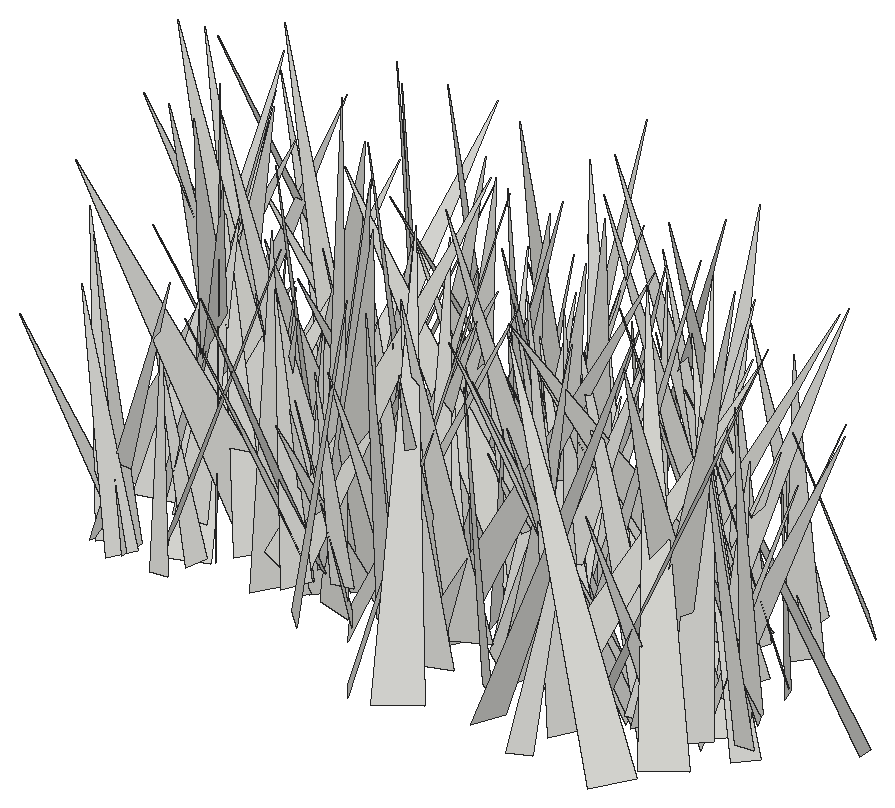
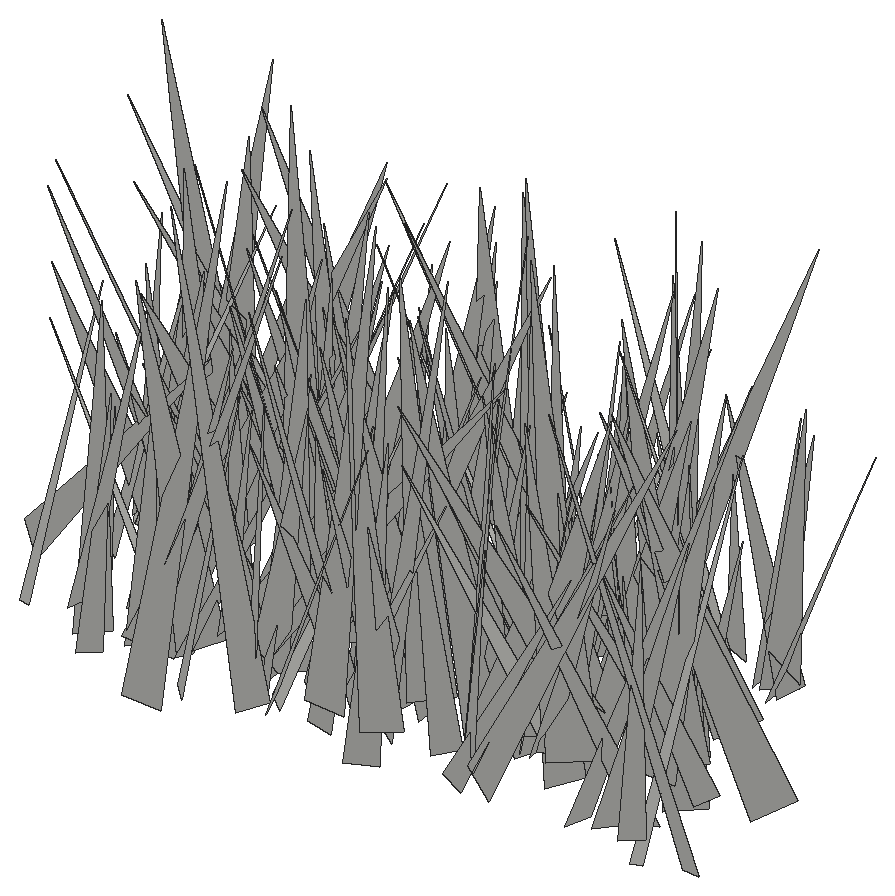
# SketchUp Ruby script. Lengths in inches.
U = 1.inch
M = Sketchup.active_model
def pt(a) = Geom::Point3d.new(a.map { |v| v * U })
def face(e, loops, mat)
  f = e.add_face(loops[0].map { |a| pt(a) })
  loops[1..].each { |l| e.add_face(l.map { |a| pt(a) }).erase! }
  f.material = f.back_material = mat if mat
  f
end
# faces: each face lists its corners as indices into pts; further lists are holes
def faces(e, pts, list, mat = nil) = list.each { |f| face(e, (f[0].is_a?(Array) ? f : [f]).map { |l| l.map { |i| pts[i] } }, mat) }
# xy, xz, yz: faces in a plane at the given z, y or x. An outline is a flat list of corners, or four numbers for a rectangle; further outlines are holes
def ring(l) = l.size == 4 ? [[l[0], l[1]], [l[2], l[1]], [l[2], l[3]], [l[0], l[3]]] : l.each_slice(2).to_a
def flat(e, list, mat, &to3) = list.each { |f| face(e, (f[0].is_a?(Array) ? f : [f]).map { |l| ring(l).map { |u, v| to3.(u, v) } }, mat) }
def xy(e, z, list, mat = nil) = flat(e, list, mat) { |x, y| [x, y, z] }
def xz(e, y, list, mat = nil) = flat(e, list, mat) { |x, z| [x, y, z] }
def yz(e, x, list, mat = nil) = flat(e, list, mat) { |y, z| [x, y, z] }
def lines(e, pts, list) = list.each { |a, b| e.add_line(pt(pts[a]), pt(pts[b])) }
# prism: a flat outline (further loops are holes) pulled along v
def prism(e, loops, v, mat = nil)
  f = face(e, loops, mat); d = Geom::Vector3d.new(v.map { |x| x * U })
  f.pushpull(f.normal.samedirection?(d) ? d.length : -d.length)
end
def box(e, o, s, mat = nil) = prism(e, [[o, [o[0] + s[0], o[1], o[2]], [o[0] + s[0], o[1] + s[1], o[2]], [o[0], o[1] + s[1], o[2]]]], [0, 0, s[2]], mat)
def at(x, y, z, deg = 0) = Geom::Transformation.translation(pt([x, y, z])) * Geom::Transformation.rotation(ORIGIN, Z_AXIS, deg.degrees)
def axes(o, x, y, z) = Geom::Transformation.new([*x, 0, *y, 0, *z, 0, *pt(o).to_a, 1])
def part(name) = M.definitions.add(name)
# library, detail: a bought-in or finely detailed component or shape, given as its bounding box
def library(name, o, s) = part(name).tap { |d| box(d.entities, o, s) }
def detail(e, o, s) = box(e.add_group.entities, o, s)
def put(e, d, t, mat = nil) = e.add_instance(d, t).tap { |i| i.material = mat if mat }
def group(e, t, mat = nil) = e.add_group.tap { |g| g.transformation = t; g.material = mat if mat }.entities
root = M.entities
c1 = part("fur_instance\#9")
p = [[0.8125,0,1.79],[0.67,-0.02,1.48],[0,-0.11,0],[0,0.11,0]]
faces(c1.entities,p,[[0,1,2,3]])
put(root,c1,axes([135.27,59.21,-27.1],[-3.78872,6.01371,0.63065],[5.87535,3.48538,2.06137],[-1.42923,-1.61377,6.8022]))
put(root,c1,axes([131.91,58.89,-27.1],[-3.54385,2.2292,0.7922],[1.93522,3.55225,-1.33876],[1.36083,0.75365,3.96686]))
put(root,c1,axes([127.14,58.92,-27.1],[-5.31707,5.30249,0.96243],[5.27581,5.39738,-0.58989],[1.09932,-0.2564,7.48596]))
put(root,c1,axes([113.87,62.25,-27.1],[-4.07009,-1.55263,0.42821],[-1.43545,4.0247,0.94922],[0.73043,-0.7422,4.25151]))
put(root,c1,axes([114.78,60.99,-27.1],[-3.50037,2.65675,1.28484],[2.86731,3.53339,0.50538],[0.69832,-1.19104,4.36526]))
put(root,c1,axes([129.83,59.96,-27.1],[7.1879,-0.3196,1.18159],[-0.53762,-7.14753,1.33717],[-1.09967,1.40532,7.06966]))
put(root,c1,axes([126.66,61.46,-27.1],[0.55696,-4.64877,2.01019],[-4.98122,-0.86859,-0.62855],[-0.91614,1.89648,4.63963]))
put(root,c1,axes([134.92,62.44,-27.1],[0.09538,-4.31944,0.7575],[-4.29634,-0.24392,-0.84995],[-0.8791,0.72346,4.23607]))
put(root,c1,axes([128.7,61.33,-27.1],[2.49829,3.83803,2.30798],[4.11646,-3.0089,0.54773],[-1.76409,-1.58579,4.54664]))
put(root,c1,axes([115.36,62.45,-27.1],[6.89965,2.05968,0.48381],[2.11498,-6.67017,-1.76557],[0.05673,-1.82978,6.98071]))
put(root,c1,axes([113.62,61.57,-27.1],[4.85484,-0.93426,0.93937],[-1.01134,-4.91828,0.33525],[-0.85583,0.51221,4.93253]))
put(root,c1,axes([116.41,60.75,-27.1],[0.5097,3.85536,0.87755],[3.83119,-0.70034,0.85159],[-0.9777,-0.73445,3.79452]))
put(root,c1,axes([114.83,61.41,-27.1],[-5.03296,-0.41167,1.23228],[-0.52474,5.15421,-0.42127],[1.18855,0.5323,5.03216]))
put(root,c1,axes([119.65,64.26,-27.1],[-2.17037,-5.72704,0.1674],[-5.69455,2.17595,0.61228],[0.63178,-0.0613,6.09382]))
put(root,c1,axes([125.42,58.64,-27.1],[6.25178,5.32919,0.93445],[4.93149,-6.20008,2.36594],[-2.22574,1.23164,7.86685]))
put(root,c1,axes([119.88,63.85,-27.1],[-3.92471,-3.72483,0.22437],[-3.66233,3.90735,0.80501],[0.71557,-0.43166,5.35067]))
put(root,c1,axes([114.01,61.63,-27.1],[3.17127,-3.30736,3.04126],[-3.82504,-3.9403,-0.2965],[-2.35731,1.94429,4.57249]))
put(root,c1,axes([121.37,61.125,-27.1],[3.52114,3.87417,1.40413],[3.91467,-3.72163,0.45161],[-1.28689,-0.72073,5.21571]))
put(root,c1,axes([123.875,62.54,-27.1],[-1.84582,-5.09705,1.94608],[-5.40108,1.99766,0.10933],[0.77171,1.78987,5.41987]))
put(root,c1,axes([124.68,64.16,-28.22],[4.57924,-4.33247,0.58798],[-4.22206,-4.60304,-1.03525],[-1.13589,-0.35667,6.21836]))
put(root,c1,axes([117.24,64.87,-27.1],[-7.12654,1.94071,2.81889],[3.04033,6.57978,3.15641],[1.57127,-3.9294,6.67765]))
put(root,c1,axes([126.48,63.34,-27.1],[1.47343,-6.07806,1.78682],[-6.21699,-1.74005,-0.79238],[-1.21846,1.52838,6.20371]))
put(root,c1,axes([131.23,63.52,-27.1],[-0.49716,-5.04462,0.80589],[-5.07325,0.39247,-0.67299],[-0.59982,0.86174,5.02418]))
put(root,c1,axes([132.2,60.74,-27.1],[-6.81045,0.95525,0.6863],[0.79996,6.71798,-1.4123],[0.86231,1.31226,6.73054]))
put(root,c1,axes([134.09,64.75,-27.1],[5.76412,-4.56343,1.38579],[-4.26746,-5.90574,-1.69745],[-2.12934,-0.51736,7.15322]))
put(root,c1,axes([135.99,60.79,-27.1],[-2.86004,7.00076,0.77945],[7.00763,2.7424,1.08181],[-0.71502,-1.12544,7.48466]))
put(root,c1,axes([131.6,64.83,-28.22],[-6.83596,-2.73328,0.53057],[-2.58478,6.75268,1.48423],[1.035,-1.18879,7.21098]))
put(root,c1,axes([132.64,61.36,-27.1],[7.12948,2.21776,0.41944],[2.17259,-7.11974,0.71624],[-0.61174,0.56098,7.43203]))
put(root,c1,axes([131.6875,64.74,-28.22],[-5.72076,-3.26575,0.35826],[-3.1922,5.6955,0.94426],[0.77675,-0.64548,6.51924]))
put(root,c1,axes([133.92,62.98,-27.1],[7.67247,-2.21843,2.0813],[-2.41925,-7.8734,0.52613],[-1.84403,1.09916,7.96941]))
put(root,c1,axes([116.74,63.1,-27.1],[-5.8561,-4.67693,3.47291],[-5.12361,6.47844,0.0849],[2.77191,2.09401,7.49403]))
put(root,c1,axes([120.1,62.8,-27.1],[-4.33048,1.8912,1.2808],[1.94847,4.49129,-0.04381],[1.19187,-0.47097,4.72523]))
put(root,c1,axes([123.3,64.1,-27.1],[0.25989,-4.12749,1.06746],[-4.12688,-0.51192,-0.97467],[-1.06982,0.97209,4.01917]))
put(root,c1,axes([121.22,63.62,-27.1],[0.17752,-3.57602,1.3313],[-3.7929,-0.31113,-0.32997],[-0.41733,1.30655,3.56518]))
put(root,c1,axes([119.8,64.51,-28.22],[2.18541,-3.04998,0.78828],[-3.02604,-2.29919,-0.50659],[-0.87571,0.3334,3.71777]))
put(root,c1,axes([120.69,65.35,-28.22],[1.51991,-3.61395,0.26794],[-3.4425,-1.53065,-1.11749],[-1.13207,-0.1975,3.75792]))
put(root,c1,axes([115.63,63.53,-28.22],[-3.79892,0.58903,0.61511],[0.5899,3.84804,-0.04166],[0.61427,-0.05255,3.84409]))
put(root,c1,axes([127.8125,63.81,-28.22],[6.14943,-1.42717,1.61929],[-1.52874,-6.3314,0.22535],[-1.52376,0.59247,6.30885]))
put(root,c1,axes([120.11,64.93,-27.1],[7.47084,-2.00529,1.5784],[-1.88161,-7.62701,-0.78379],[-1.72397,-0.36551,7.69548]))
put(root,c1,axes([119.8,65.61,-28.22],[6.18232,-5.30847,0.7026],[-5.32058,-6.21081,-0.10875],[-0.60412,0.37485,8.14795]))
put(root,c1,axes([121.6,63.51,-28.22],[5.9079,4.20697,0.32991],[4.15488,-5.69984,-1.72033],[0.73785,-1.5887,7.04573]))
put(root,c1,axes([121.75,63.53,-28.22],[-3.12705,-1.8127,0.50032],[-1.87769,2.95706,-1.02213],[-0.10232,1.13341,3.46693]))
put(root,c1,axes([118.37,63.7,-28.22],[-5.0872,2.66073,2.45988],[2.85923,5.55214,-0.09239],[2.22604,-1.05084,5.74025]))
put(root,c1,axes([137.01,63.43,-27.1],[-2.00481,-4.221,2.16779],[-4.72189,1.54205,-1.3643],[-0.46899,2.51807,4.46932]))
put(root,c1,axes([130.46,62.32,-27.1],[1.42855,6.69806,0.59183],[6.31436,-1.12829,-2.47201],[2.31152,-1.05735,6.38701]))
put(root,c1,axes([124.61,63.72,-28.22],[-2.01026,5.06538,1.49078],[5.275,1.85579,0.80751],[-0.23431,-1.67916,5.38954]))
put(root,c1,axes([125.57,62.92,-27.1],[7.23014,-2.66142,0.8801],[-2.79977,-6.73645,2.62947],[0.1379,2.76941,7.24182]))
put(root,c1,axes([133.41,63.68,-28.22],[-6.69944,1.03913,0.45559],[1.00559,6.70154,-0.49804],[0.5255,0.42362,6.76123]))
put(root,c1,axes([130.05,64,-27.1],[-5.84783,-0.54956,0.92386],[-0.66437,5.86496,-0.71656],[0.84507,0.80798,5.82972]))
put(root,c1,axes([135.58,62.65,-27.1],[-6.65914,2.85732,1.17721],[2.6023,6.69305,-1.52492],[1.66678,0.96593,7.084]))
put(root,c1,axes([115.02,63.98,-27.1],[-0.99114,4.85366,1.48422],[5.00835,1.18049,-0.51592],[0.82303,-1.33855,4.92689]))
put(root,c1,axes([119.22,63.28,-27.1],[1.74287,7.71217,1.36191],[7.45298,-1.20484,-2.71503],[2.4053,-1.85492,7.42588]))
put(root,c1,axes([127.33,64.32,-28.22],[5.24089,-0.83273,1.62957],[-1.05437,-5.41429,0.62423],[-1.49573,0.89885,5.2698]))
put(root,c1,axes([127.91,64.1,-28.22],[0.11042,6.13884,2.00494],[6.14565,0.51615,-1.91884],[1.98398,-1.94051,5.83229]))
put(root,c1,axes([119.18,65.49,-27.1],[-7.26017,0.65472,1.63239],[0.85,7.37598,0.82207],[1.53976,-0.9847,7.24313]))
put(root,c1,axes([136.2,64.83,-27.1],[-5.05567,-0.39861,1.84756],[-0.46846,5.37567,-0.1221],[1.83109,0.27472,5.06989]))
put(root,c1,axes([113.81,67.375,-27.1],[7.57168,-2.77915,1.4038],[-2.39268,-7.55557,-2.05259],[-1.99233,-1.48808,7.80006]))
put(root,c1,axes([117.86,63.4375,-27.1],[-5.44212,1.96061,0.21811],[1.90755,5.39324,-0.88463],[0.50284,0.7598,5.71648]))
put(root,c1,axes([130.01,64.14,-27.1],[-5.54219,0.95074,1.40051],[0.80502,5.69802,-0.68242],[1.48905,0.4581,5.58158]))
put(root,c1,axes([112.8,67.72,-28.22],[8.00988,-2.00577,0.3429],[-1.833,-7.71682,-2.32157],[-0.88363,-2.17404,7.92412]))
put(root,c1,axes([124.8125,63.58,-27.1],[-0.46142,6.00885,1.03301],[6.04976,0.32253,0.82618],[-0.75742,-1.08443,5.96964]))
put(root,c1,axes([120.74,63.85,-28.22],[2.99088,7.34321,2.70362],[7.47912,-3.53374,1.32409],[-2.30112,-1.94104,7.81761]))
put(root,c1,axes([136.26,65.15,-27.1],[-5.87124,-3.56524,0.53214],[-3.58838,5.68376,-1.51131],[-0.34307,1.5651,6.70063]))
put(root,c1,axes([130.94,63.56,-27.1],[-1.18961,5.30841,0.21099],[4.92708,1.02155,2.07828],[-1.98686,-0.64508,5.02744]))
put(root,c1,axes([127,66.19,-27.1],[2.07554,-6.96607,1.71735],[-7.11885,-1.77704,1.39545],[0.89291,2.02467,7.13349]))
put(root,c1,axes([122.99,65.53,-27.1],[-6.35073,-3.49942,2.22612],[-3.7296,6.59945,-0.26567],[1.81428,1.31702,7.24617]))
put(root,c1,axes([134.78,65.42,-27.1],[-0.53957,3.97433,2.02364],[4.38519,0.84425,-0.48882],[0.81275,-1.91664,3.98089]))
put(root,c1,axes([114.22,63.33,-27.1],[5.15399,5.0376,1.12923],[4.93282,-5.27609,1.02292],[-1.5231,-0.04087,7.13405]))
put(root,c1,axes([124.59,64.875,-27.1],[-2.6188,2.85202,1.01974],[2.95253,2.70449,0.01846],[0.67563,-0.76402,3.87193]))
put(root,c1,axes([136.3,64.375,-28.22],[-1.36293,4.52681,0.55653],[4.38086,1.13777,1.47406],[-1.26877,-0.93423,4.49185]))
put(root,c1,axes([119.51,64.17,-28.22],[-4.10668,0.43412,1.0008],[0.12519,4.05996,-1.24738],[1.0837,1.17608,3.93666]))
put(root,c1,axes([134.34,66.25,-28.22],[1.7038,-4.78318,1.39426],[-4.94528,-1.80274,-0.14134],[-0.60574,1.26373,5.0756]))
put(root,c1,axes([129.3,64.13,-27.1],[-2.23012,3.65012,0.738],[3.54975,2.34365,-0.86487],[1.12574,-0.15918,4.18913]))
put(root,c1,axes([116.7,65.43,-27.1],[2.33806,3.32528,1.40975],[3.5899,-2.32407,-0.47188],[-0.3968,-1.43269,4.03749]))
put(root,c1,axes([121.08,66.53,-27.1],[-0.06945,-5.66946,1.63507],[-5.27402,0.7929,2.5253],[2.64594,1.43164,5.07647]))
put(root,c1,axes([121.36,65.04,-28.22],[3.29943,5.39851,1.49465],[5.593,-3.07886,-1.22601],[0.31023,-1.9081,6.20701]))
put(root,c1,axes([134.49,64.36,-28.22],[3.07177,3.42083,0.35758],[3.42072,-3.08846,0.16062],[-0.35863,-0.15826,4.59478]))
put(root,c1,axes([129.5,64.56,-28.22],[5.42391,5.6075,1.42758],[5.74422,-5.4537,-0.40246],[-0.69711,-1.3092,7.79108]))
put(root,c1,axes([116.05,66.67,-27.1],[-0.58442,-4.16845,1.10453],[-3.96593,0.95723,1.51414],[1.69333,0.80327,3.92746]))
put(root,c1,axes([117.41,65.62,-28.22],[1.80806,-4.3936,1.6396],[-4.55829,-1.23367,1.72079],[1.10181,2.10605,4.4285]))
put(root,c1,axes([127.69,66.6,-27.1],[-1.28539,6.13898,3.44989],[6.89976,0.39684,1.86462],[-1.40785,-3.66012,5.98853]))
put(root,c1,axes([114,65.36,-28.22],[-4.83531,-1.63891,2.39644],[-2.01972,5.24312,-0.48946],[2.08559,1.27782,5.08199]))
put(root,c1,axes([125.01,66.39,-28.22],[3.69206,0.52175,1.19179],[0.74035,-3.79133,-0.63373],[-1.0698,-0.8231,3.6745]))
put(root,c1,axes([130.55,65.91,-28.22],[-4.50374,-2.5863,0.2222],[-2.55985,4.35118,-1.23954],[-0.43072,1.18335,5.04343]))
put(root,c1,axes([131.88,70.02,-28.22],[4.91107,-6.51993,1.1851],[-5.42781,-4.80392,-3.93621],[-3.80168,-1.5638,7.15082]))
put(root,c1,axes([122.79,65.05,-28.22],[-5.72971,0.10944,0.75393],[-0.02545,5.68949,-1.01935],[0.7614,1.01378,5.63937]))
put(root,c1,axes([127.63,67.52,-27.1],[3.37968,-7.43588,1.46776],[-7.57694,-3.27406,0.85991],[0.19143,1.6903,8.12251]))
put(root,c1,axes([125.64,67.29,-27.1],[-6.93796,2.79801,1.11968],[3.01121,6.55067,2.28891],[0.12298,-2.54512,7.12215]))
put(root,c1,axes([116.3,66.67,-27.1],[-4.3642,6.37446,3.0679],[7.06974,4.05938,1.62241],[0.25406,-3.46117,7.553]))
put(root,c1,axes([126.7,64.33,-28.22],[4.48947,6.23838,0.89691],[6.27438,-4.52789,0.08708],[-0.59503,-0.67674,7.68539]))
put(root,c1,axes([117.66,67.28,-28.22],[-4.21383,-5.23135,2.06774],[-5.35043,4.52497,0.54449],[1.7365,1.24763,6.69529]))
put(root,c1,axes([135.3,67.56,-27.1],[-3.21192,-3.98216,0.77509],[-3.98629,3.28152,0.34045],[0.75355,0.38579,5.10471]))
put(root,c1,axes([135.09,65.3,-28.22],[-3.60307,5.2202,0.86904],[5.28801,3.51043,0.83765],[-0.20649,-1.18922,6.28736]))
put(root,c1,axes([127.23,67.4375,-28.22],[0.6602,-3.48398,0.63366],[-3.31771,-0.83389,-1.12823],[-1.23791,0.37685,3.36171]))
put(root,c1,axes([115.35,63.5,-28.22],[-5.02723,4.35262,0.08247],[4.19421,4.87628,-1.68986],[1.1665,1.22544,6.43138]))
put(root,c1,axes([133.55,62.85,-27.1],[-6.0414,2.82747,0.77084],[2.14541,5.47009,-3.25002],[1.99649,2.67784,5.82499]))
put(root,c1,axes([124.2,66.33,-28.22],[2.78644,2.89477,1.9564],[3.12581,-3.18339,0.25829],[-1.56092,-1.20736,4.00964]))
put(root,c1,axes([125.74,67.13,-28.22],[2.18387,-4.44969,1.85832],[-4.59717,-2.53702,-0.67228],[-1.45572,1.33648,4.91091]))
put(root,c1,axes([115.99,66.53,-27.1],[3.13173,2.6382,1.54856],[2.8558,-3.31576,-0.12654],[-1.0966,-1.10068,4.0929]))
put(root,c1,axes([128.23,64.74,-28.22],[-3.94538,2.89092,1.6801],[2.22143,4.20848,-2.02488],[2.49909,0.82308,4.45234]))
put(root,c1,axes([113.33,67.16,-27.1],[4.2743,-5.66959,1.70794],[-5.91958,-4.14155,1.06631],[-0.14077,2.00854,7.01974]))
put(root,c1,axes([126.37,65.36,-28.22],[0.1573,5.82785,1.1486],[5.93788,-0.12389,-0.18455],[0.15705,-1.15268,5.82705]))
put(root,c1,axes([126,66.07,-28.22],[6.01682,-1.89651,1.60783],[-2.22,-5.99358,1.23799],[-1.11958,1.69241,6.18597]))
put(root,c1,axes([117.75,68.37,-27.1],[3.73697,-5.4189,0.58942],[-5.45085,-3.71358,0.41766],[0.01126,0.72231,6.56925]))
put(root,c1,axes([116.83,69.03,-27.1],[4.42124,-3.27,0.9733],[-2.9097,-4.44582,-1.71927],[-1.78153,-0.85401,5.22344]))
put(root,c1,axes([133.94,66.33,-27.1],[4.38543,-2.43855,0.87514],[-2.59033,-4.09309,1.5752],[0.05089,1.80126,4.76417]))
put(root,c1,axes([117.72,64.85,-27.1],[-0.98442,7.82804,0.7856],[7.24103,0.59195,3.17514],[-3.07617,-1.11168,7.22258]))
put(root,c1,axes([110.66,66.1,-28.22],[5.79439,-3.93356,1.43708],[-4.17619,-5.2444,2.48372],[0.31237,2.85246,6.54821]))
put(root,c1,axes([133.47,68.29,-28.22],[3.25434,-3.10316,1.28908],[-2.93626,-3.49873,-1.00964],[-1.63392,0.10675,4.38189]))
put(root,c1,axes([130.6,66.34,-27.1],[4.59981,5.90875,0.46757],[5.722,-4.27232,-2.30133],[1.54616,-1.76752,7.12569]))
put(root,c1,axes([113.44,64.375,-27.1],[-5.30404,4.85737,1.41696],[4.30663,5.41145,-2.42976],[2.65607,0.92563,6.76928]))
put(root,c1,axes([113.57,68.29,-27.1],[0.65749,-6.30029,1.7132],[-6.47052,-0.85883,-0.67511],[-0.87239,1.62165,6.29842]))
put(root,c1,axes([124.79,66.99,-27.1],[2.82445,3.52777,0.66946],[3.53756,-2.58781,-1.2883],[0.61561,-1.31488,4.33162]))
put(root,c1,axes([118.61,67.71,-28.22],[3.69144,-5.31541,0.62902],[-5.0613,-3.21782,2.51095],[1.74141,1.9152,5.96452]))
put(root,c1,axes([130.69,69.77,-28.22],[-6.06549,-1.51995,0.44377],[-1.27134,5.72216,2.22212],[0.94386,-2.06007,5.84487]))
put(root,c1,axes([116.1,69.0625,-27.1],[3.30529,-7.09092,0.75642],[-7.06387,-3.14139,1.41833],[0.97724,1.27626,7.69379]))
put(root,c1,axes([119.27,69.54,-27.1],[0.9036,-5.03288,0.01557],[-4.93923,-0.88981,-0.97923],[-0.96652,-0.158,5.01871]))
put(root,c1,axes([124.92,68.01,-27.1],[-5.6933,-0.47947,0.5538],[-0.44449,5.71072,0.37467],[0.58224,-0.32872,5.70116]))
put(root,c1,axes([118.86,67.68,-27.1],[4.80209,-1.99507,1.20954],[-2.10711,-4.89697,0.2883],[-1.00169,0.73669,5.19204]))
put(root,c1,axes([132.38,67.375,-27.1],[0.51441,-3.71167,1.78135],[-3.92489,0.09986,1.3415],[1.24297,1.85145,3.49879]))
put(root,c1,axes([138.84,67.02,-28.22],[-3.79929,-4.93063,0.76728],[-4.2284,2.66909,-3.78564],[-2.64961,2.81057,4.94112]))
put(root,c1,axes([115.47,66.8,-28.22],[0.89714,3.83975,1.01573],[3.88067,-1.06922,0.61438],[-0.84607,-0.83267,3.89501]))
put(root,c1,axes([132.69,66.51,-27.1],[2.40606,6.39383,1.08481],[6.38564,-2.13376,-1.58675],[1.13207,-1.55339,6.64473]))
put(root,c1,axes([114.79,66.14,-27.1],[1.15422,4.7345,0.08294],[4.6056,-1.10261,-1.15208],[1.10037,-0.35121,4.73502]))
put(root,c1,axes([116.48,68.03,-28.22],[1.60896,-4.17155,1.4473],[-4.41412,-1.4813,0.63763],[0.1098,1.57772,4.42538]))
put(root,c1,axes([111.86,71.29,-28.22],[-3.50557,-5.51536,0.11612],[-4.95597,3.20905,2.80393],[2.42302,-1.41579,5.90306]))
put(root,c1,axes([131.35,66.12,-28.22],[1.15539,6.15443,1.22459],[6.01284,-1.44203,1.57415],[-1.79512,-0.86897,6.06086]))
put(root,c1,axes([125.16,67.89,-28.22],[2.89079,5.81329,3.19782],[6.3896,-3.37876,0.3661],[-1.787,-2.67707,6.48205]))
put(root,c1,axes([114.93,70.3,-28.22],[-7.42684,-1.75978,1.28146],[-1.36577,7.3143,2.12899],[1.69519,-1.81689,7.32954]))
put(root,c1,axes([118.68,66.6,-27.1],[4.79219,0.94532,0.41054],[0.81575,-4.67249,1.23678],[-0.62985,1.14081,4.72537]))
put(root,c1,axes([128.04,66.61,-27.1],[5.65388,1.0827,1.74004],[0.6959,-5.81697,1.3583],[-1.92762,1.07564,5.59407]))
put(root,c1,axes([121.86,68.75,-27.1],[5.17414,-4.36417,1.70527],[-4.54977,-5.28673,0.27499],[-1.1196,1.31532,6.76329]))
put(root,c1,axes([127.16,67.16,-27.1],[-1.66344,3.87519,0.54462],[3.91265,1.65754,0.1564],[0.06977,-0.56232,4.21422]))
put(root,c1,axes([132.44,69.11,-28.22],[-7.92829,-1.68885,1.19775],[-1.65667,8.01779,0.33921],[1.24187,-0.08605,8.09907]))
put(root,c1,axes([129.25,68.96,-27.1],[-2.36065,-3.34559,0.0438],[-3.13879,2.19578,-1.44709],[-1.15883,0.86782,3.83035]))
put(root,c1,axes([111.43,68.43,-27.1],[2.74116,-2.85153,0.16279],[-2.64199,-2.44575,1.64616],[1.08517,1.2485,3.59657]))
put(root,c1,axes([129.14,68.99,-28.22],[-4.42248,-6.55022,0.11235],[-5.68971,3.77318,-3.9833],[-3.24733,2.30957,6.8262]))
put(root,c1,axes([122.66,67.6,-28.22],[6.83211,0.09479,1.62922],[-0.11306,-6.96812,0.87954],[-1.62805,0.88169,6.77592]))
put(root,c1,axes([120.33,67.91,-28.22],[6.64236,-2.17739,2.19825],[-2.53423,-6.81539,0.90685],[-1.77512,1.5823,6.93106]))
put(root,c1,axes([124.69,70.6875,-28.22],[-2.64137,-6.46023,1.04071],[-6.35863,2.79897,1.23619],[1.54452,0.47506,6.86901]))
put(root,c1,axes([126.42,69.04,-28.22],[-2.99975,-3.60869,1.08185],[-3.74003,3.01886,-0.30041],[0.45307,1.02732,4.68304]))
put(root,c1,axes([117.92,69.35,-27.1],[-3.40624,-2.616,1.08161],[-2.59295,3.56228,0.44999],[1.13575,0.28715,4.27123]))
put(root,c1,axes([127.63,69.76,-28.22],[-2.72161,-4.19987,1.18368],[-4.18397,2.90781,0.69726],[1.23872,0.59401,4.95579]))
put(root,c1,axes([126.68,70.28,-28.22],[-3.4454,-3.89131,0.03074],[-3.88746,3.44363,0.20759],[0.17579,-0.11462,5.19326]))
put(root,c1,axes([116.73,68.68,-28.22],[5.24676,-2.59436,1.90695],[-2.83441,-5.4512,0.38233],[-1.5275,1.20389,5.84064]))
put(root,c1,axes([120.6875,69.49,-28.22],[3.98619,-2.41358,0.43201],[-2.42835,-4.00018,0.05811],[-0.33929,0.27366,4.65958]))
put(root,c1,axes([129.46,67.46,-27.1],[0.97735,4.73028,0.44464],[4.65378,-0.86171,-1.06216],[0.95682,-0.64061,4.71196]))
put(root,c1,axes([134.76,68.35,-28.22],[-3.3024,-1.44134,1.34219],[-1.74105,3.36144,-0.674],[0.92071,1.18661,3.53964]))
put(root,c1,axes([132.86,68.59,-27.1],[4.03846,2.29721,0.25382],[2.30928,-3.98992,-0.63131],[0.09403,-0.6739,4.60302]))
put(root,c1,axes([119.08,67.28,-27.1],[-0.71343,7.62578,1.29035],[7.14993,0.15622,3.02994],[-2.94889,-1.46615,7.03427]))
put(root,c1,axes([123.24,69.45,-28.22],[-4.43723,-6.45792,2.6794],[-6.95056,4.4181,-0.86196],[0.75734,2.71083,7.78786]))
put(root,c1,axes([127.76,68.51,-28.22],[-4.29093,5.93832,1.73067],[6.14946,4.32229,0.41585],[0.66564,-1.65078,7.31456]))
put(root,c1,axes([135.29,71.77,-27.1],[-2.98193,-4.15353,0.46379],[-3.81224,2.9367,1.78925],[1.71281,-0.69483,4.78981]))
put(root,c1,axes([118.04,71.17,-27.1],[-5.4355,-1.48683,0.1699],[-1.41481,5.31415,1.24191],[0.48767,-1.15472,5.49664]))
put(root,c1,axes([113.99,69.95,-28.22],[-4.9541,1.83691,1.27432],[2.05779,4.95762,0.85363],[0.87385,-1.26054,5.21428]))
put(root,c1,axes([132.2,70.01,-28.22],[3.95695,-1.9726,1.7752],[-1.97238,-4.31833,-0.40205],[-1.77544,0.40099,4.40306]))
put(root,c1,axes([129.49,69.16,-27.1],[-4.34694,-0.07841,1.0456],[-0.20123,4.43859,-0.5037],[1.02905,0.53671,4.31837]))
put(root,c1,axes([124.08,71.19,-27.1],[-1.04012,-7.65192,1.88155],[-7.84849,1.17518,0.4406],[0.70237,1.80029,7.70971]))
put(root,c1,axes([117.26,66.82,-27.1],[-0.93463,7.10607,0.24964],[6.82555,0.96718,-1.97702],[1.99262,0.02006,6.88921]))
put(root,c1,axes([123.86,70.32,-27.1],[-2.53875,-3.10556,0.31926],[-3.0835,2.42999,-0.88252],[-0.48832,0.80145,3.91291]))
put(root,c1,axes([127.74,69.34,-28.22],[3.90442,0.1948,1.09665],[0.0575,-4.02752,0.51071],[-1.11233,0.47558,3.87577]))
put(root,c1,axes([117.39,67.82,-28.22],[5.65943,2.62486,0.30549],[2.50558,-5.55953,1.3513],[-0.8398,1.10185,6.0904]))
put(root,c1,axes([119.4,70.84,-28.22],[-0.92246,-4.02488,0.49642],[-3.83236,0.69867,-1.45667],[-1.32631,0.78053,3.86377]))
put(root,c1,axes([133.76,70.37,-28.22],[4.08918,-3.36848,1.98263],[-3.52303,-4.41912,-0.24183],[-1.69286,1.05996,5.29241]))
put(root,c1,axes([122.26,71.67,-28.22],[2.722,-4.21365,0.18087],[-4.20663,-2.72794,-0.24377],[-0.30292,0.01939,5.01046]))
put(root,c1,axes([121.82,71.24,-27.1],[2.30675,-6.01681,0.97122],[-6.03702,-2.11321,1.24701],[0.83643,1.34116,6.32203]))
put(root,c1,axes([125.18,69,-27.1],[4.28943,0.41298,0.87796],[0.18379,-4.25331,1.1028],[-0.95267,1.03894,4.16576]))
put(root,c1,axes([127.97,69.125,-28.22],[-4.785,3.6619,0.62252],[3.69492,4.79647,0.18627],[0.38032,-0.52686,6.02254]))
put(root,c1,axes([129.88,72.83,-28.22],[-1.4202,-8.16889,0.91065],[-8.13373,1.52988,1.03868],[1.18423,0.71114,8.22611]))
put(root,c1,axes([120.39,68.88,-28.22],[-6.74078,-2.87477,2.26806],[-3.46071,6.55422,-1.97791],[1.19661,2.76122,7.05622]))
put(root,c1,axes([133.97,70.71,-27.1],[-5.16901,0.01394,1.37798],[0.15537,5.32107,0.52899],[1.36927,-0.55116,5.14189]))
put(root,c1,axes([117.46,68.76,-27.1],[-6.47288,0.26814,0.01301],[0.25719,6.28405,-1.55397],[0.07694,1.55212,6.2893]))
put(root,c1,axes([131.41,69.74,-27.1],[-5.82181,0.2065,0.70872],[0.14567,5.84473,-0.50632],[0.72368,0.48471,5.80343]))
put(root,c1,axes([123.96,68.77,-27.1],[4.21835,1.12148,1.8478],[0.48542,-4.44001,1.58659],[-2.10629,1.22277,4.06632]))
put(root,c1,axes([111.69,71.74,-27.1],[3.7269,-2.05729,0.24824],[-1.97365,-3.67974,-0.86491],[-0.63149,-0.64103,4.16823]))
put(root,c1,axes([126.77,70.4,-28.22],[-5.1041,-1.8904,0.52095],[-1.9461,5.06157,-0.70004],[0.24022,0.83889,5.39772]))
put(root,c1,axes([110.26,70.66,-28.22],[4.54413,5.8348,1.67226],[5.93472,-3.83302,-2.75273],[1.27295,-2.95864,6.86415]))
put(root,c1,axes([131.12,70.875,-27.1],[-7.49054,-0.65717,0.9559],[-0.61994,7.54719,0.33069],[0.98046,-0.24861,7.51203]))
put(root,c1,axes([133.06,71.39,-28.22],[3.43553,-2.13589,0.95207],[-2.02418,-3.56342,-0.68999],[-1.17096,-0.10667,3.98608]))
put(root,c1,axes([118.9375,70.55,-27.1],[-4.32305,-4.69404,2.5219],[-5.10648,4.57733,-0.23372],[1.52244,2.02405,6.37716]))
put(root,c1,axes([123.45,68.29,-28.22],[-4.67511,2.29396,0.21165],[2.12082,4.47274,-1.63107],[0.89953,1.37696,4.94555]))
put(root,c1,axes([130.56,69.04,-28.22],[5.55139,-3.03279,3.66915],[-4.09539,-5.91606,1.30628],[-2.42657,3.04644,6.18946]))
put(root,c1,axes([129.37,71.6,-28.22],[-3.40896,-3.60182,1.17644],[-3.63778,3.55381,0.3393],[1.06005,0.61272,4.94762]))
put(root,c1,axes([117.51,71.92,-27.1],[-3.5976,-6.50533,0.64098],[-6.34012,3.29439,-2.15004],[-1.59153,1.58132,7.11613]))
put(root,c1,axes([113.2,69.19,-28.22],[0.65579,5.75921,0.77226],[5.58682,-0.41126,-1.67728],[1.5976,-0.92592,5.54845]))
put(root,c1,axes([126.53,71.71,-27.1],[2.79226,2.81825,2.22878],[3.51982,-2.71249,-0.9798],[-0.72174,-2.32521,3.84438]))
put(root,c1,axes([124.5,69,-28.22],[3.66563,6.83822,1.35122],[6.90712,-3.76874,0.33492],[-0.93742,-1.02919,7.75151]))
put(root,c1,axes([125.8,72.52,-27.1],[7.87771,-0.03675,0.30438],[0.03502,-7.66773,-1.83222],[-0.30459,-1.83219,7.66177]))
